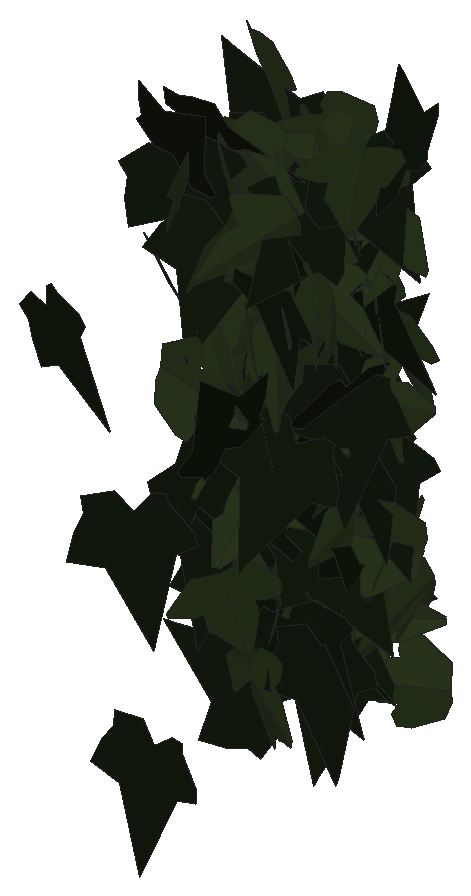
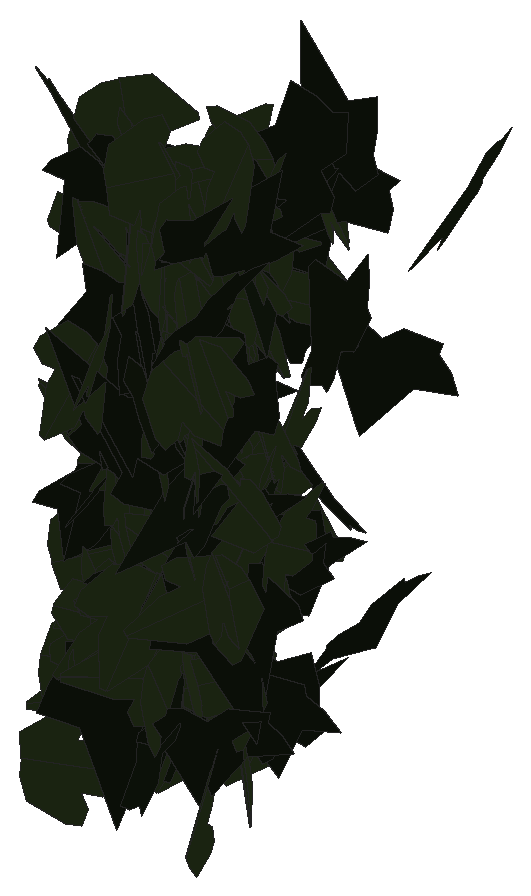
# SketchUp Ruby script. Lengths in inches.
U = 1.inch
M = Sketchup.active_model
def pt(a) = Geom::Point3d.new(a.map { |v| v * U })
def face(e, loops, mat)
  f = e.add_face(loops[0].map { |a| pt(a) })
  loops[1..].each { |l| e.add_face(l.map { |a| pt(a) }).erase! }
  f.material = f.back_material = mat if mat
  f
end
# faces: each face lists its corners as indices into pts; further lists are holes
def faces(e, pts, list, mat = nil) = list.each { |f| face(e, (f[0].is_a?(Array) ? f : [f]).map { |l| l.map { |i| pts[i] } }, mat) }
# xy, xz, yz: faces in a plane at the given z, y or x. An outline is a flat list of corners, or four numbers for a rectangle; further outlines are holes
def ring(l) = l.size == 4 ? [[l[0], l[1]], [l[2], l[1]], [l[2], l[3]], [l[0], l[3]]] : l.each_slice(2).to_a
def flat(e, list, mat, &to3) = list.each { |f| face(e, (f[0].is_a?(Array) ? f : [f]).map { |l| ring(l).map { |u, v| to3.(u, v) } }, mat) }
def xy(e, z, list, mat = nil) = flat(e, list, mat) { |x, y| [x, y, z] }
def xz(e, y, list, mat = nil) = flat(e, list, mat) { |x, z| [x, y, z] }
def yz(e, x, list, mat = nil) = flat(e, list, mat) { |y, z| [x, y, z] }
def lines(e, pts, list) = list.each { |a, b| e.add_line(pt(pts[a]), pt(pts[b])) }
# prism: a flat outline (further loops are holes) pulled along v
def prism(e, loops, v, mat = nil)
  f = face(e, loops, mat); d = Geom::Vector3d.new(v.map { |x| x * U })
  f.pushpull(f.normal.samedirection?(d) ? d.length : -d.length)
end
def box(e, o, s, mat = nil) = prism(e, [[o, [o[0] + s[0], o[1], o[2]], [o[0] + s[0], o[1] + s[1], o[2]], [o[0], o[1] + s[1], o[2]]]], [0, 0, s[2]], mat)
def at(x, y, z, deg = 0) = Geom::Transformation.translation(pt([x, y, z])) * Geom::Transformation.rotation(ORIGIN, Z_AXIS, deg.degrees)
def axes(o, x, y, z) = Geom::Transformation.new([*x, 0, *y, 0, *z, 0, *pt(o).to_a, 1])
def part(name) = M.definitions.add(name)
# library, detail: a bought-in or finely detailed component or shape, given as its bounding box
def library(name, o, s) = part(name).tap { |d| box(d.entities, o, s) }
def detail(e, o, s) = box(e.add_group.entities, o, s)
def put(e, d, t, mat = nil) = e.add_instance(d, t).tap { |i| i.material = mat if mat }
def group(e, t, mat = nil) = e.add_group.tap { |g| g.transformation = t; g.material = mat if mat }.entities
root = M.entities
M.materials.add("efeu1").color = [18, 25, 13]
M.materials.add("efeu2").color = [43, 57, 29]
c1 = part("ivyleaf_9")
p = [[1.54,2.16,1.25],[1.36,2.04,1.19],[-0.21,0.99,0.68],[-0.71,1.11,0.82],[-0.85,0.86,0.67],[-0.8,0.17,0.21],
  [-0.9,-0.01,0.1],[-0.67,-0.16,-0.02],[-0.08,-0.08,-0.05],[-0.03,-0.6,-0.4],[0.65,-0.88,-0.66],[0.83,-0.6,-0.49],
  [1.29,-0.42,-0.43],[1.8125,-0.07,-0.26],[1.21,0.44,0.15]]
faces(c1.entities,p,[[0,1,2,3,4,5,6,7,8,9,10,11,12,13,14]],"efeu1")
c2 = part("ivyleaf_10")
p = [[0,0.5,-0.03],[-0.0625,2.02,-0.43],[-0.19,2.01,-0.46],[-0.54,1.05,-0.29],[-0.52,0.625,-0.18],[-0.83,0.76,-0.28],
  [-1.16,0.64,-0.33],[-1.15,0.33,-0.24],[-0.77,-0.39,0.02],[-0.3,-0.51,0.16],[0.04,-0.48,0.23],[-0.02,2.01,-0.4375],
  [-0.06,2.01,-0.43],[0.04,-0.49,0.23],[0.67,-0.49,0.14],[1.38,0.36,-0.2],[1.375,0.51,-0.24],[0.81,0.65,-0.19],
  [0.62,0.59,-0.15],[0.6,1.09,-0.28],[0.5,1.23,-0.31]]
faces(c2.entities,p,[[0,1,2,3,4,5,6,7,8,9,10],[11,12,0,13,14,15,16,17,18,19,20]],"efeu2")
put(root,c1,axes([24.24,222.82,211.61],[0.07704,-0.23025,0.4371],[0.20054,-0.38972,-0.24063],[0.4515,0.21238,0.0323]))
put(root,c2,axes([24.5,224.09,214.06],[-0.40617,0.27057,-0.10871],[0.09061,-0.06006,-0.48804],[-0.27715,-0.41616,-0.00025]))
put(root,c2,axes([24.28,224.1,210.25],[0.3566,-0.08406,-0.34025],[0.33942,-0.03811,0.36516],[-0.08732,-0.49141,0.02988]))
put(root,c1,axes([24.39,220.52,212.33],[0.32465,-0.362,-0.11643],[-0.07422,0.08983,-0.48623],[0.37295,0.33299,0.00459]))
put(root,c2,axes([24.7,223.15,210.36],[-0.13639,0.48079,0.01558],[-0.01378,-0.02009,0.49941],[0.48084,0.1358,0.01873]))
put(root,c2,axes([24.52,223.34,209.56],[-0.03341,-0.26133,0.42496],[0.22759,-0.38699,-0.22009],[0.44394,0.17873,0.14481]))
put(root,c2,axes([24.59,222.66,213.29],[0.24494,-0.39357,0.18738],[0.10044,-0.15819,-0.46356],[0.42417,0.26473,0.00157]))
put(root,c2,axes([24.64,224.08,209.53],[0.09176,-0.46549,0.1578],[0.06734,-0.14711,-0.4731],[0.48687,0.10808,0.03569]))
put(root,c1,axes([24.88,224.03,212.92],[-0.38137,-0.32178,0.03183],[0.05738,-0.01891,0.49634],[-0.31822,0.38223,0.05136]))
put(root,c1,axes([24.8,223.84,209.18],[0.21336,0.31598,-0.32348],[-0.18048,-0.26845,-0.38126],[-0.41462,0.27945,-0.0005]))
put(root,c1,axes([24.45,222.59,213.4],[-0.1419,-0.04155,0.47764],[0.29357,-0.40135,0.0523],[0.37905,0.29528,0.1383]))
put(root,c2,axes([24.61,223.52,211.07],[0.43545,-0.22023,0.10902],[0.09465,-0.05439,-0.48794],[0.22677,0.44558,-0.00568]))
put(root,c1,axes([24.49,222.61,213.32],[-0.10674,-0.26146,-0.41261],[0.21175,0.35583,-0.28026],[0.44019,-0.23457,0.03477]))
put(root,c1,axes([24.68,223.71,211.58],[0.44065,0.05975,-0.22861],[-0.22646,-0.03122,-0.44468],[-0.06741,0.49543,-0.00045]))
put(root,c1,axes([24.72,223.51,208.02],[-0.36435,-0.25747,-0.22575],[0.18316,0.13198,-0.44613],[0.28931,-0.40779,-0.00186]))
put(root,c2,axes([24.86,223.57,207.67],[0.23313,-0.37577,-0.23334],[-0.10298,0.2104,-0.44173],[0.43017,0.25402,0.02071]))
put(root,c1,axes([24.7,224.0625,210.05],[-0.15963,-0.47259,0.03427],[-0.00844,-0.03333,-0.49882],[0.47376,-0.15983,0.00267]))
put(root,c1,axes([24.37,223.02,213.57],[0.35982,-0.13425,0.32016],[0.30548,-0.09664,-0.38385],[0.16495,0.47184,0.01247]))
put(root,c1,axes([24.65,224.45,212.5],[-0.0173,-0.48355,0.12601],[-0.01438,-0.12555,-0.48377],[0.49949,-0.02036,-0.00957]))
put(root,c1,axes([24.67,224.27,207.98],[-0.22486,-0.37727,-0.23896],[0.13911,0.19506,-0.43886],[0.42437,-0.26385,0.01724]))
put(root,c2,axes([24.86,223.04,213.34],[-0.25075,0.41519,0.12144],[-0.05887,0.10631,-0.48501],[-0.42856,-0.25752,-0.00443]))
put(root,c2,axes([24.96,224.37,211.68],[-0.08508,-0.39613,0.29299],[-0.05207,-0.28843,-0.40509],[0.48995,-0.09944,0.00783]))
put(root,c2,axes([24.74,224.35,206.77],[-0.14471,0.18045,0.44328],[0.28449,-0.33998,0.23126],[0.38487,0.31915,-0.00428]))
put(root,c1,axes([25.15,223.01,212.4],[-0.12364,0.36769,0.31546],[-0.09764,0.29998,-0.38791],[-0.47453,-0.15753,-0.00237]))
put(root,c2,axes([24.6,223.9375,208.39],[-0.2614,0.05895,-0.42213],[0.40756,-0.11037,-0.26779],[-0.12475,-0.48409,0.00965]))
put(root,c2,axes([24.96,223.9,210.89],[0.04786,-0.47186,-0.1583],[0.00335,0.15933,-0.47392],[0.49769,0.04431,0.01841]))
put(root,c1,axes([24.6875,223.7,209.69],[0.07901,-0.35216,0.34603],[0.06594,-0.33977,-0.36084],[0.48929,0.10266,-0.00725]))
put(root,c2,axes([24.67,224.04,209.31],[-0.19833,-0.13931,-0.43733],[0.4016,0.17799,-0.23882],[0.22222,-0.446,0.0413]))
put(root,c1,axes([25.15,222.16,209.53],[-0.45876,0.18837,-0.06366],[-0.06274,0.01477,0.49583],[0.18868,0.46292,0.01008]))
put(root,c2,axes([25.09,223.82,213.24],[-0.33052,-0.35477,0.12203],[-0.07287,-0.09882,-0.48469],[0.36803,-0.33818,0.01362]))
put(root,c2,axes([25.05,223.74,211.1875],[-0.09935,-0.47144,-0.13368],[0.02613,0.13111,-0.4818],[0.48933,-0.10272,-0.00141]))
put(root,c2,axes([25.03,224.02,211.73],[0.4863,-0.06103,-0.09895],[-0.09691,0.02224,-0.49001],[0.06421,0.49576,0.0098]))
put(root,c1,axes([24.89,223.85,213.15],[-0.06958,-0.48905,-0.0774],[0.01747,0.07568,-0.49393],[0.49483,-0.07144,0.00656]))
put(root,c1,axes([24.94,222.8125,208.95],[-0.12737,-0.48349,0.0042],[0.0018,-0.00482,-0.49997],[0.4835,-0.12735,0.00297]))
put(root,c1,axes([24.83,224.07,210.48],[0.46689,-0.17302,-0.04557],[-0.04254,0.01635,-0.49792],[0.17379,0.46883,0.00054]))
put(root,c2,axes([25.21,223.16,212.11],[0.43074,-0.12291,-0.22216],[-0.2143,0.05863,-0.44793],[0.13616,0.4811,-0.00217]))
put(root,c2,axes([25.15,223.98,212.24],[0.15957,-0.45931,-0.11649],[-0.04677,0.10705,-0.48616],[0.47154,0.16605,-0.0088]))
put(root,c1,axes([24.81,223.05,207.38],[-0.11591,-0.02079,0.48594],[0.40055,-0.28745,0.08325],[0.27591,0.40858,0.08329]))
put(root,c2,axes([25.15,222.61,212.61],[0.00938,-0.45928,-0.19742],[0.02902,0.19762,-0.45837],[0.49907,-0.00285,0.03036]))
put(root,c1,axes([25.09,222.66,212.59],[-0.21408,-0.45175,-0.00964],[0.00246,0.0095,-0.4999],[0.45185,-0.21409,-0.00184]))
put(root,c2,axes([25.18,223.84,208.37],[0.20454,-0.43761,0.12909],[0.05815,-0.11531,-0.48303],[0.45253,0.21262,0.00373]))
put(root,c2,axes([25.42,222.75,211.06],[-0.01668,0.0167,-0.49944],[-0.21469,0.45101,0.02225],[0.45126,0.21519,-0.00787]))
put(root,c2,axes([25.06,224,209.98],[0.12983,-0.29955,0.37871],[0.25461,-0.29073,-0.31725],[0.41026,0.27522,0.07705]))
put(root,c2,axes([25.23,224.3,208.21],[0.10323,-0.45417,0.18187],[0.07336,-0.1694,-0.46467],[0.4837,0.12262,0.03166]))
put(root,c2,axes([25.62,223.77,213.125],[-0.19283,0.00823,0.46125],[-0.45677,0.06661,-0.19215],[-0.06461,-0.49547,-0.01817]))
put(root,c2,axes([25.28,223.6,212.6],[-0.3943,-0.27736,-0.13266],[0.10413,0.08252,-0.48202],[0.28929,-0.40775,-0.00731]))
put(root,c2,axes([25.09,223.4,212.38],[-0.36607,0.03007,-0.33925],[0.33657,-0.04428,-0.3671],[-0.05212,-0.49713,0.01217]))
put(root,c1,axes([25.58,222.82,206.92],[-0.22129,-0.43884,-0.09191],[-0.04053,-0.0825,0.49148],[-0.44653,0.22497,0.00094]))
put(root,c2,axes([25.41,223.45,211.66],[-0.01054,-0.35028,-0.35664],[-0.00654,0.35679,-0.35023],[0.49985,-0.00272,-0.0121]))
put(root,c2,axes([25.06,223.125,213.48],[-0.22294,0.05032,-0.44471],[0.39845,-0.20392,-0.22283],[-0.2038,-0.45374,0.05083]))
put(root,c1,axes([25.16,222.74,208.78],[-0.22507,-0.0538,0.44323],[0.43825,-0.12147,0.2078],[0.08532,0.48203,0.10183]))
put(root,c2,axes([25.3125,223.31,207.56],[-0.10822,-0.32125,-0.36754],[0.16151,0.3317,-0.33748],[0.46066,-0.19177,0.03198]))
put(root,c2,axes([25.45,223.14,207],[-0.16787,-0.28303,-0.37645],[-0.1231,-0.35939,0.32509],[-0.45461,0.20183,0.05097]))
put(root,c2,axes([25.53,223.44,208.36],[0.13832,-0.27409,-0.39464],[-0.09853,0.38576,-0.30246],[0.47027,0.16144,0.05271]))
put(root,c1,axes([25.1,224.46,207.62],[0.2652,-0.08292,-0.41568],[0.3932,-0.13501,0.27779],[-0.15831,-0.47423,-0.0064]))
put(root,c1,axes([25.625,223.57,211.77],[-0.01031,0.37784,-0.32731],[-0.03314,-0.32718,-0.37664],[-0.49879,0.01393,0.03178]))
put(root,c2,axes([25.65,222.87,208.23],[0.02253,-0.10304,-0.48875],[-0.18792,0.45155,-0.10386],[0.46279,0.18837,-0.01838]))
put(root,c1,axes([25.18,223.49,211.3125],[0.10299,-0.26162,0.41346],[0.14617,-0.38678,-0.28114],[0.46694,0.17877,-0.00319]))
put(root,c2,axes([25.13,222.75,208.65],[-0.038,0.02982,-0.49766],[0.41605,-0.27311,-0.04813],[-0.2747,-0.41776,-0.00405]))
put(root,c2,axes([25.75,224.07,213.45],[-0.03915,-0.02703,-0.49773],[-0.40722,-0.28619,0.04757],[-0.28747,0.4091,0.0004]))
put(root,c2,axes([25.32,224.27,212.4375],[0.06876,-0.24672,-0.42942],[0.12461,-0.41098,0.25607],[-0.47932,-0.14223,0.00497]))
put(root,c2,axes([25.51,222.65,209.66],[0.39298,0.26083,-0.16594],[-0.13975,-0.08951,-0.47165],[-0.27575,0.41708,0.00255]))
put(root,c2,axes([25.53,223.67,210.83],[-0.04802,-0.48407,-0.11564],[0.02066,0.11414,-0.48636],[0.49726,-0.05149,0.00904]))
put(root,c2,axes([25.19,223.83,209.23],[-0.19324,-0.08046,0.45408],[0.42461,0.16103,0.20923],[-0.17991,0.46647,0.0061]))
put(root,c1,axes([25.65,224,211.34],[-0.34574,0.27108,-0.23871],[0.19095,-0.14331,-0.43932],[-0.30659,-0.39494,-0.00443]))
put(root,c1,axes([25.15,223.76,208.01],[0.15035,-0.17251,0.44456],[0.35279,-0.27338,-0.2254],[0.32083,0.38145,0.03952]))
put(root,c2,axes([25.16,221.74,211.22],[0.06997,0.02571,0.49441],[0.48487,0.09734,-0.07368],[-0.10004,0.48976,-0.01131]))
put(root,c2,axes([25.58,222.68,210.24],[-0.42641,0.23609,0.1115],[0.09499,-0.0586,0.48738],[0.2432,0.43684,0.00512]))
put(root,c1,axes([25.27,223.88,210.26],[-0.07365,0.0053,0.49452],[0.48347,-0.10442,0.07313],[0.10405,0.48895,0.01026]))
put(root,c2,axes([25.38,223.92,211.58],[0.24233,-0.20839,0.38452],[0.31011,-0.22811,-0.31906],[0.3084,0.39312,0.0187]))
put(root,c2,axes([25.625,223.09,212.3],[-0.02915,0.12191,0.48403],[0.08436,-0.47668,0.12514],[0.49197,0.08896,0.00722]))
put(root,c2,axes([25.63,224.06,208.93],[-0.47195,-0.10514,-0.12731],[0.12431,0.02747,-0.48352],[0.10867,-0.48805,0.00021]))
put(root,c2,axes([25.81,222.64,212.95],[-0.03471,-0.2139,0.4506],[-0.11326,-0.43651,-0.21594],[0.48576,-0.11707,-0.01815]))
put(root,c1,axes([25.55,220.54,210.1875],[-0.26014,-0.27547,-0.32626],[0.21527,0.24532,-0.37878],[0.36876,-0.33754,-0.00903]))
put(root,c1,axes([25.45,223.53,212.46],[-0.0144,-0.29342,0.40459],[0.16416,-0.38508,-0.27343],[0.47206,0.12496,0.10743]))
put(root,c2,axes([25.72,221.91,208.79],[-0.32758,-0.35755,-0.12185],[0.08271,0.08947,-0.48493],[0.36858,-0.33786,0.00053]))
put(root,c2,axes([25.6,224.31,212.45],[-0.30134,0.23891,0.31955],[0.25333,-0.1948,0.38455],[0.30824,0.39366,-0.00364]))
put(root,c2,axes([25.37,223.61,212.32],[0.18014,0.0727,0.46072],[0.43898,0.14046,-0.19381],[-0.15761,0.47433,-0.01322]))
put(root,c2,axes([25.43,223.93,208.07],[0.01356,-0.00292,0.49981],[0.36216,0.34464,-0.00781],[-0.34446,0.36223,0.01146]))
put(root,c1,axes([25.62,220.77,207.22],[-0.00972,-0.49079,0.09503],[-0.00301,-0.09499,-0.49089],[0.4999,-0.01011,-0.00111]))
put(root,c2,axes([26.04,223.88,208.37],[-0.37281,-0.06485,-0.32681],[-0.32327,-0.04834,0.37836],[-0.08067,0.49341,-0.00589]))
put(root,c1,axes([26.09,223.93,212.49],[-0.46029,0.19403,0.02196],[-0.02039,0.00817,-0.49952],[-0.1942,-0.46074,0.00039]))
put(root,c1,axes([25.57,224.18,212.3],[-0.04422,-0.06899,-0.49324],[0.49563,-0.05478,-0.03677],[-0.04896,-0.49218,0.07323]))
put(root,c2,axes([25.57,222.68,209.75],[0.13088,0.07039,-0.47741],[0.44516,0.17334,0.1476],[0.18629,-0.46368,-0.01729]))
put(root,c1,axes([25.9,223.24,212.85],[-0.17892,-0.39171,0.25407],[-0.08007,-0.24231,-0.42997],[0.45998,-0.19454,0.02398]))
put(root,c1,axes([25.87,221.71,210.68],[0.15892,0.22406,0.41778],[-0.22978,-0.34901,0.27458],[0.41466,-0.27927,-0.00796]))
put(root,c1,axes([26.02,223.89,207.87],[0.15495,0.45748,-0.12922],[-0.0418,-0.12227,-0.48301],[-0.47354,0.16049,0.00036]))
put(root,c1,axes([25.54,223.78,207.32],[0.26678,-0.23712,0.35015],[0.25815,-0.23659,-0.35691],[0.33494,0.37121,-0.00381]))
put(root,c1,axes([25.67,222.77,212.08],[0.12296,-0.41986,0.24208],[0.11321,-0.21796,-0.43552],[0.47124,0.16191,0.04146]))
put(root,c2,axes([25.91,223.71,213.61],[0.46277,-0.18921,0.00679],[0.00677,-0.00137,-0.49995],[0.18921,0.46282,0.0013]))
put(root,c1,axes([25.7,224.12,210.51],[-0.17958,0.10985,0.45352],[0.39239,-0.22745,0.21046],[0.25255,0.43151,-0.00451]))
put(root,c2,axes([25.77,223.91,208.58],[-0.29067,-0.1568,-0.3754],[0.34961,0.13966,-0.32903],[0.20805,-0.45377,0.02845]))
put(root,c2,axes([25.74,222.67,211.55],[0.3542,-0.14968,0.31959],[0.28876,-0.13738,-0.38438],[0.20288,0.45686,-0.01088]))
put(root,c1,axes([25.84,223.85,208.72],[-0.03489,-0.26319,0.42369],[0.04177,-0.42478,-0.26042],[0.49703,0.01722,0.05163]))
put(root,c2,axes([26.06,223.73,209.97],[0.02512,-0.48938,-0.09939],[-0.01305,0.09884,-0.48996],[0.4992,0.02721,-0.00781]))
put(root,c1,axes([26.18,223.4,210.72],[-0.13953,0.38466,-0.28734],[0.06976,-0.27981,-0.40846],[-0.47504,-0.15408,0.02441]))
put(root,c2,axes([26.08,223.35,209.64],[0.18677,-0.45962,-0.0622],[-0.02131,0.05848,-0.49611],[0.46332,0.18796,0.00225]))
put(root,c2,axes([26.04,223.87,207.28],[-0.02286,-0.07883,0.49322],[0.10418,-0.48363,-0.07247],[0.48849,0.09945,0.03853]))
put(root,c2,axes([25.98,224.25,211.71],[-0.16495,0.4228,-0.20983],[0.07633,-0.19545,-0.45384],[-0.4658,-0.18175,-0.00007]))
put(root,c2,axes([25.79,223.43,211.84],[-0.24853,-0.01955,-0.43342],[0.41859,-0.14215,-0.23362],[-0.11409,-0.47897,0.08703]))
put(root,c1,axes([25.84,222.89,207.93],[-0.12622,-0.12938,-0.46618],[0.33831,0.3208,-0.18064],[0.34585,-0.36103,0.00656]))
put(root,c1,axes([26.13,222.56,210.35],[-0.32934,-0.37491,-0.03125],[0.02003,0.02401,-0.49902],[0.37568,-0.32995,-0.0008]))
put(root,c1,axes([26.08,223.42,207.4375],[-0.28788,-0.38531,-0.13662],[0.08457,0.10735,-0.48096],[0.39997,-0.30002,0.00336]))
put(root,c1,axes([25.94,223.35,208.8125],[0.01797,-0.37063,-0.33513],[0.12715,0.3277,-0.35559],[0.48323,-0.07244,0.10603]))
put(root,c1,axes([26.11,223.51,209.05],[0.22723,-0.39256,-0.2104],[0.16559,-0.14481,0.44901],[-0.41346,-0.27374,0.0642]))
put(root,c1,axes([26.03,223.6,209.96],[-0.00602,-0.33439,-0.37168],[0.08932,0.36501,-0.32983],[0.49192,-0.07036,0.05534]))
put(root,c2,axes([26.02,223.72,207.68],[0.00418,0.02917,0.49913],[0.23961,0.43798,-0.0276],[-0.43883,0.23943,-0.01031]))
put(root,c2,axes([25.98,222.23,207.5],[-0.07547,0.08084,-0.48762],[0.33669,-0.35272,-0.11058],[-0.36186,-0.34504,-0.0012]))
put(root,c1,axes([26.2,223.51,210.625],[-0.17216,-0.45005,-0.13348],[0.03229,0.13049,-0.48159],[0.46831,-0.17444,-0.01587]))
put(root,c2,axes([26.64,224.26,206.84],[0.00496,0.0107,0.49986],[-0.38585,-0.31782,0.01063],[0.31796,-0.38585,0.0051]))
put(root,c1,axes([26.15,223.7,213.375],[-0.06837,-0.32278,-0.37568],[0.09406,0.36388,-0.32976],[0.48629,-0.11577,0.01096]))
put(root,c1,axes([25.99,223.91,211.69],[-0.00037,0.0025,-0.49999],[0.47266,0.16307,0.00047],[0.16307,-0.47265,-0.00248]))
put(root,c2,axes([26.46,223.34,213.67],[-0.33466,-0.36367,0.0758],[-0.04713,-0.05963,-0.49419],[0.36849,-0.33792,0.00564]))
put(root,c2,axes([26.27,223.47,209.24],[-0.02687,-0.06103,0.49553],[0.18145,-0.46351,-0.04724],[0.46514,0.17729,0.04706]))
put(root,c2,axes([26.42,223.81,208.31],[0.16082,-0.25811,0.39688],[-0.1758,0.35663,0.30316],[-0.43958,-0.23705,0.02396]))
put(root,c2,axes([26.72,223.67,208.86],[-0.10019,-0.04721,-0.48758],[-0.45247,-0.18177,0.11058],[-0.1877,0.46339,-0.0063]))
put(root,c1,axes([26.1875,223.73,210.01],[0.1282,-0.4826,0.02562],[0.0082,-0.02433,-0.49934],[0.48321,0.12846,0.00167]))
put(root,c1,axes([26.27,223.73,209.8],[-0.12936,-0.3534,-0.32921],[0.09761,0.31465,-0.37612],[0.47301,-0.16157,-0.01242]))
put(root,c2,axes([26.43,223.86,212.67],[0.49246,-0.0414,-0.07594],[-0.07493,0.01504,-0.49412],[0.0432,0.49806,0.00861]))
put(root,c2,axes([26.48,224.02,208.23],[-0.09286,-0.103,0.48038],[0.02256,-0.48927,-0.10055],[0.49078,0.003,0.09552]))
put(root,c1,axes([26.28,222.88,207.75],[0.02252,-0.49343,-0.07758],[-0.00601,0.07738,-0.49394],[0.49946,0.02318,-0.00244]))
put(root,c2,axes([26.35,224.1,211.25],[-0.43372,0.19095,-0.15945],[0.1462,-0.06364,-0.47389],[-0.20127,-0.4577,-0.00063]))
put(root,c2,axes([26.21,223.07,211.92],[-0.12663,-0.07898,0.47721],[0.38212,-0.31878,0.04864],[0.29656,0.37702,0.14109]))
put(root,c1,axes([26.78,223.6875,213.59],[-0.38832,0.15152,-0.27614],[-0.25491,0.10631,0.4168],[0.18502,0.46448,-0.00531]))
put(root,c2,axes([26.51,224.19,208],[0.02841,-0.22279,0.44672],[0.05785,-0.44296,-0.22459],[0.49583,0.06444,0.00061]))
put(root,c2,axes([26.15,223.99,210.35],[0.10324,-0.06235,-0.48524],[0.43882,-0.20744,0.12002],[-0.21628,-0.45065,0.01189]))
